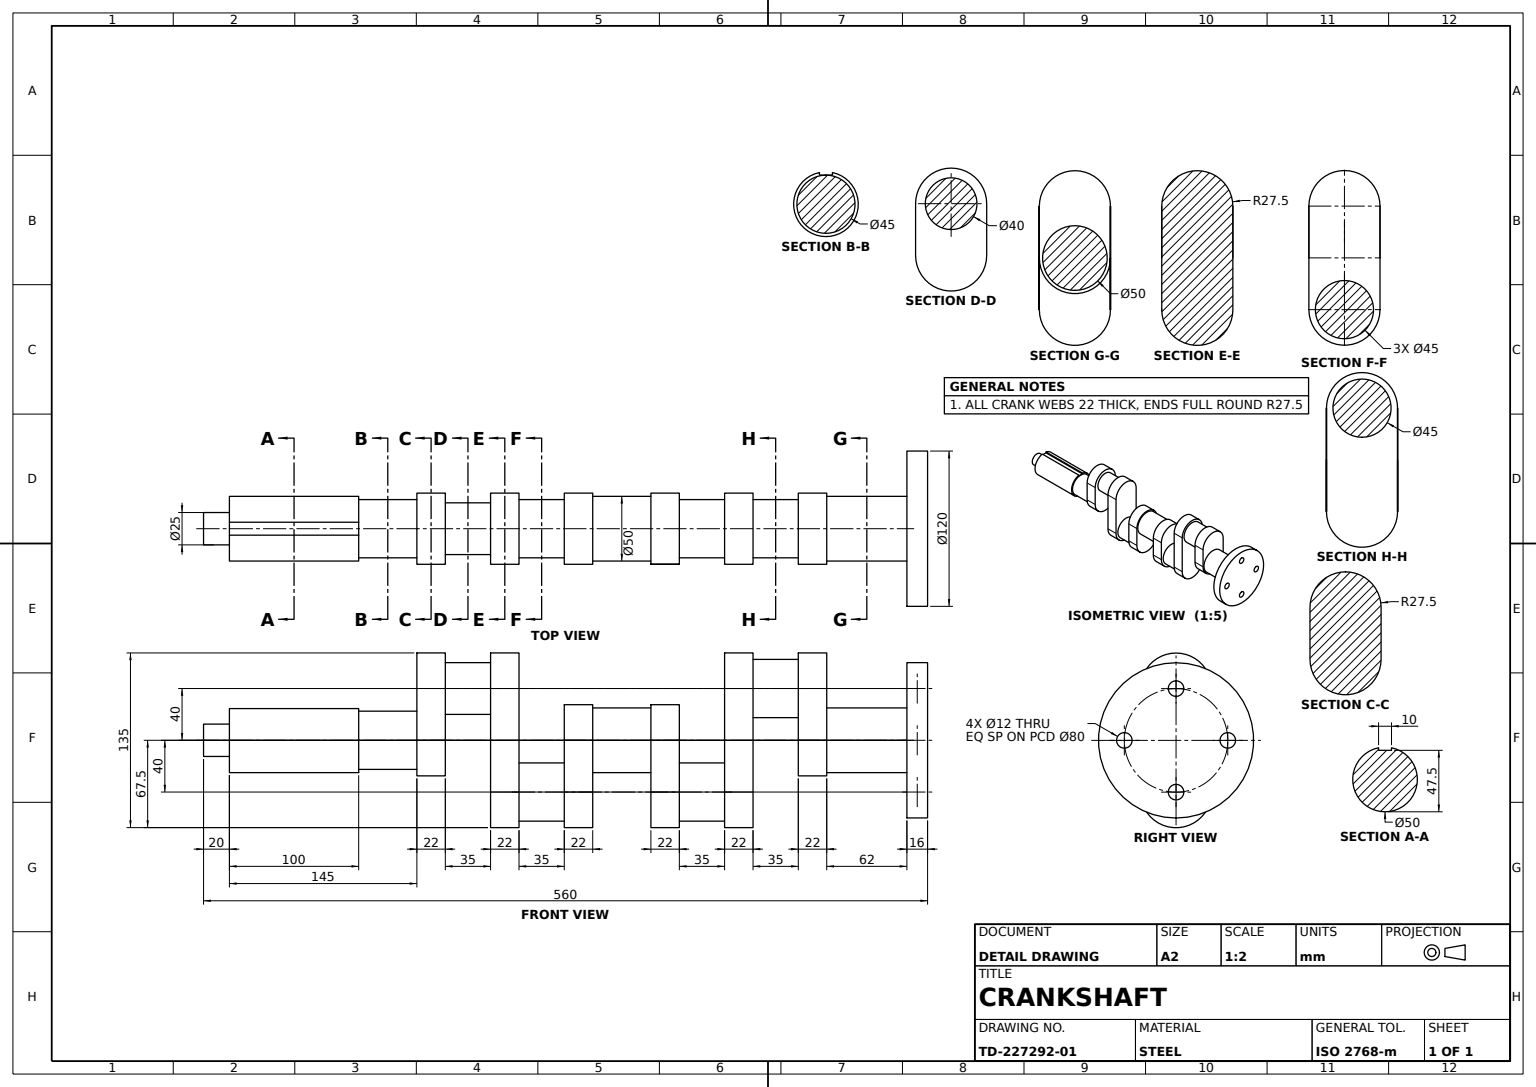
solid
v1 (-17.5,0,135)
v2 (-62.5,0,135)
e1 v1 v2 CIRCLE(AX(P(-40,0,135),D(0,0,1),D(1,0,0)),22.5)
e2 v2 v1 CIRCLE(AX(P(-40,0,135),D(0,0,1),D(1,0,0)),22.5)
v3 (-40,27.5,135)
v4 (-67.5,0,135)
e3 v3 v4 CIRCLE(AX(P(-40,0,135),D(0,0,1),D(1,0,0)),27.5)
v5 (40,27.5,135)
e4 v5 v3 LINE
v6 (40,-27.5,135)
e5 v6 v5 CIRCLE(AX(P(40,0,135),D(0,0,1),D(1,0,0)),27.5)
v7 (-40,-27.5,135)
e6 v7 v6 LINE
e7 v4 v7 CIRCLE(AX(P(-40,0,135),D(0,0,1),D(1,0,0)),27.5)
face PLANE(AX(P(-40,0,135),D(0,0,1),D(1,0,0))) rev [e1 e2] [-e3 -e4 -e5 -e6 -e7]
v8 (-6,40,0)
v9 (-6,40,16)
e8 v8 v9 LINE
v10 (6,40,16)
e9 v9 v10 CIRCLE(AX(P(0,40,16),D(0,0,1),D(1,0,0)),6)
v11 (6,40,0)
e10 v11 v10 LINE
e11 v8 v11 CIRCLE(AX(P(0,40,0),D(0,0,1),D(1,0,0)),6)
face CYL(AX(P(0,40,-4),D(0,0,1),D(1,0,0)),6) rev [e8 e9 -e10 -e11]
v12 (17.5,0,281)
v13 (62.5,0,281)
e12 v12 v13 CIRCLE(AX(P(40,0,281),D(0,0,1),D(1,0,0)),22.5)
e13 v13 v12 CIRCLE(AX(P(40,0,281),D(0,0,1),D(1,0,0)),22.5)
v14 (40,27.5,281)
v15 (0,27.5,281)
e14 v14 v15 LINE
v16 (-27.5,0,281)
e15 v15 v16 CIRCLE(AX(P(0,0,281),D(0,0,1),D(1,0,0)),27.5)
v17 (0,-27.5,281)
e16 v16 v17 CIRCLE(AX(P(0,0,281),D(0,0,1),D(1,0,0)),27.5)
v18 (40,-27.5,281)
e17 v17 v18 LINE
e18 v18 v14 CIRCLE(AX(P(40,0,281),D(0,0,1),D(1,0,0)),27.5)
face PLANE(AX(P(0,0,281),D(0,0,1),D(1,0,0))) [-e12 -e13] [e14 e15 e16 e17 e18]
v19 (12.5,0,540)
v20 (-12.5,0,540)
e19 v19 v20 CIRCLE(AX(P(0,0,540),D(0,0,1),D(1,0,0)),12.5)
e20 v20 v19 CIRCLE(AX(P(0,0,540),D(0,0,1),D(1,0,0)),12.5)
v21 (25,0,540)
v22 (-24.494897,5,540)
e21 v21 v22 CIRCLE(AX(P(0,0,540),D(0,0,1),D(1,0,0)),25)
v23 (-22.5,5,540)
e22 v23 v22 LINE
v24 (-22.5,-5,540)
e23 v24 v23 LINE
v25 (-24.494897,-5,540)
e24 v25 v24 LINE
e25 v25 v21 CIRCLE(AX(P(0,0,540),D(0,0,1),D(1,0,0)),25)
face PLANE(AX(P(0,0,540),D(0,0,1),D(1,0,0))) [-e19 -e20] [e21 -e22 -e23 -e24 e25]
v26 (40,27.5,338)
v27 (40,27.5,316)
e26 v26 v27 LINE
v28 (40,-27.5,338)
e27 v28 v26 CIRCLE(AX(P(40,0,338),D(0,0,1),D(1,0,0)),27.5)
v29 (40,-27.5,316)
e28 v28 v29 LINE
e29 v29 v27 CIRCLE(AX(P(40,0,316),D(0,0,1),D(1,0,0)),27.5)
face CYL(AX(P(40,0,338),D(0,0,-1),D(-1,0,0)),27.5) [-e26 -e27 e28 e29]
v30 (62.5,0,192)
v31 (62.5,0,157)
e30 v30 v31 LINE
v32 (17.5,0,192)
e31 v32 v30 CIRCLE(AX(P(40,0,192),D(0,0,1),D(1,0,0)),22.5)
v33 (17.5,0,157)
e32 v32 v33 LINE
e33 v33 v31 CIRCLE(AX(P(40,0,157),D(0,0,1),D(1,0,0)),22.5)
face CYL(AX(P(40,0,192),D(0,0,-1),D(-1,0,0)),22.5) [-e30 -e31 e32 e33]
v34 (12.5,0,560)
e34 v34 v19 LINE
v35 (-12.5,0,560)
e35 v35 v34 CIRCLE(AX(P(0,0,560),D(0,0,1),D(1,0,0)),12.5)
e36 v35 v20 LINE
face CYL(AX(P(0,0,560),D(0,0,-1),D(-1,0,0)),12.5) [e20 -e34 -e35 e36]
v36 (25,0,78)
v37 (-25,0,78)
e37 v36 v37 CIRCLE(AX(P(0,0,78),D(0,0,1),D(1,0,0)),25)
v38 (25,0,16)
e38 v36 v38 LINE
v39 (-25,0,16)
e39 v38 v39 CIRCLE(AX(P(0,0,16),D(0,0,1),D(1,0,0)),25)
e40 v37 v39 LINE
face CYL(AX(P(0,0,78),D(0,0,-1),D(-1,0,0)),25) [-e37 e38 e39 -e40]
v40 (-67.5,0,157)
e41 v40 v4 LINE
v41 (-40,27.5,157)
e42 v41 v40 CIRCLE(AX(P(-40,0,157),D(0,0,1),D(1,0,0)),27.5)
e43 v41 v3 LINE
face CYL(AX(P(-40,0,157),D(0,0,-1),D(-1,0,0)),27.5) [-e41 -e42 e43 e3]
v42 (-20,0,373)
v43 (-20,0,338)
e44 v42 v43 LINE
v44 (-60,0,338)
e45 v43 v44 CIRCLE(AX(P(-40,0,338),D(0,0,1),D(1,0,0)),20)
v45 (-60,0,373)
e46 v45 v44 LINE
e47 v42 v45 CIRCLE(AX(P(-40,0,373),D(0,0,1),D(1,0,0)),20)
face CYL(AX(P(-40,0,373),D(0,0,-1),D(-1,0,0)),20) [e44 e45 -e46 -e47]
v46 (-24.494897,-5,440)
e48 v46 v25 LINE
v47 (25,0,440)
e49 v46 v47 CIRCLE(AX(P(0,0,440),D(0,0,1),D(1,0,0)),25)
e50 v47 v21 LINE
face CYL(AX(P(0,0,440),D(0,0,1),D(1,0,0)),25) [-e25 -e48 e49 e50]
e51 v11 v8 CIRCLE(AX(P(0,40,0),D(0,0,1),D(1,0,0)),6)
e52 v10 v9 CIRCLE(AX(P(0,40,16),D(0,0,1),D(1,0,0)),6)
face CYL(AX(P(0,40,-4),D(0,0,1),D(1,0,0)),6) rev [-e8 -e51 e10 e52]
v48 (22.5,0,440)
v49 (-22.5,0,440)
e53 v48 v49 CIRCLE(AX(P(0,0,440),D(0,0,1),D(1,0,0)),22.5)
v50 (-22.5,5,440)
e54 v49 v50 LINE
v51 (-24.494897,5,440)
e55 v50 v51 LINE
e56 v47 v51 CIRCLE(AX(P(0,0,440),D(0,0,1),D(1,0,0)),25)
v52 (-22.5,-5,440)
e57 v46 v52 LINE
e58 v52 v49 LINE
e59 v49 v48 CIRCLE(AX(P(0,0,440),D(0,0,1),D(1,0,0)),22.5)
face PLANE(AX(P(0,0,440),D(0,0,1),D(1,0,0))) rev [e53 e54 e55 -e56 -e49 e57 e58 e59]
v53 (62.5,0,316)
e60 v53 v13 LINE
v54 (17.5,0,316)
e61 v54 v12 LINE
e62 v53 v54 CIRCLE(AX(P(40,0,316),D(0,0,1),D(1,0,0)),22.5)
face CYL(AX(P(40,0,316),D(0,0,-1),D(-1,0,0)),22.5) [e60 e13 -e61 -e62]
v55 (-40,27.5,338)
e63 v26 v55 LINE
v56 (-40,27.5,316)
e64 v27 v56 LINE
e65 v55 v56 LINE
face PLANE(AX(P(40,27.5,338),D(0,-1,0),D(1,0,0))) rev [-e63 e26 e64 -e65]
e66 v31 v33 CIRCLE(AX(P(40,0,157),D(0,0,1),D(1,0,0)),22.5)
e67 v30 v32 CIRCLE(AX(P(40,0,192),D(0,0,1),D(1,0,0)),22.5)
face CYL(AX(P(40,0,192),D(0,0,-1),D(-1,0,0)),22.5) [e30 e66 -e32 -e67]
v57 (0,27.5,395)
v58 (0,27.5,373)
e68 v57 v58 LINE
v59 (-40,27.5,373)
e69 v58 v59 LINE
v60 (-40,27.5,395)
e70 v60 v59 LINE
e71 v57 v60 LINE
face PLANE(AX(P(-40,27.5,395),D(0,-1,0),D(0,0,-1))) rev [e68 e69 -e70 -e71]
v61 (40,-27.5,157)
e72 v61 v6 LINE
v62 (40,27.5,157)
e73 v62 v5 LINE
e74 v61 v62 CIRCLE(AX(P(40,0,157),D(0,0,1),D(1,0,0)),27.5)
face CYL(AX(P(40,0,157),D(0,0,-1),D(-1,0,0)),27.5) [e72 e5 -e73 -e74]
e75 v50 v23 LINE
e76 v51 v22 LINE
face PLANE(AX(P(-24.494897,5,440),D(0,1,0),D(0,0,1))) rev [-e55 e75 e22 -e76]
v63 (-60,0,16)
v64 (60,0,16)
e77 v63 v64 CIRCLE(AX(P(0,0,16),D(0,0,1),D(1,0,0)),60)
v65 (-60,0,0)
e78 v63 v65 LINE
v66 (60,0,0)
e79 v65 v66 CIRCLE(AX(P(0,0,0),D(0,0,1),D(1,0,0)),60)
e80 v64 v66 LINE
face CYL(AX(P(0,0,16),D(0,0,-1),D(-1,0,0)),60) [-e77 e78 e79 -e80]
v67 (0,-27.5,214)
v68 (0,-27.5,192)
e81 v67 v68 LINE
v69 (40,-27.5,192)
e82 v68 v69 LINE
v70 (40,-27.5,214)
e83 v70 v69 LINE
e84 v67 v70 LINE
face PLANE(AX(P(40,-27.5,214),D(0,1,0),D(-1,0,0))) rev [e81 e82 -e83 -e84]
v71 (40,27.5,192)
e85 v69 v71 CIRCLE(AX(P(40,0,192),D(0,0,1),D(1,0,0)),27.5)
v72 (-27.5,0,192)
e86 v72 v68 CIRCLE(AX(P(0,0,192),D(0,0,1),D(1,0,0)),27.5)
v73 (0,27.5,192)
e87 v73 v72 CIRCLE(AX(P(0,0,192),D(0,0,1),D(1,0,0)),27.5)
e88 v71 v73 LINE
face PLANE(AX(P(40,0,192),D(0,0,1),D(1,0,0))) rev [e67 e31] [-e85 -e82 -e86 -e87 -e88]
v74 (-22.5,0,395)
e89 v49 v74 LINE
v75 (22.5,0,395)
e90 v74 v75 CIRCLE(AX(P(0,0,395),D(0,0,1),D(1,0,0)),22.5)
e91 v48 v75 LINE
face CYL(AX(P(0,0,540),D(0,0,-1),D(-1,0,0)),22.5) [e89 e90 -e91 -e59]
v76 (-6,-40,0)
v77 (-6,-40,16)
e92 v76 v77 LINE
v78 (6,-40,16)
e93 v77 v78 CIRCLE(AX(P(0,-40,16),D(0,0,1),D(1,0,0)),6)
v79 (6,-40,0)
e94 v79 v78 LINE
e95 v76 v79 CIRCLE(AX(P(0,-40,0),D(0,0,1),D(1,0,0)),6)
face CYL(AX(P(0,-40,-4),D(0,0,1),D(1,0,0)),6) rev [e92 e93 -e94 -e95]
v80 (-25,0,214)
v81 (25,0,214)
e96 v80 v81 CIRCLE(AX(P(0,0,214),D(0,0,1),D(1,0,0)),25)
v82 (25,0,259)
e97 v82 v81 LINE
v83 (-25,0,259)
e98 v83 v82 CIRCLE(AX(P(0,0,259),D(0,0,1),D(1,0,0)),25)
e99 v83 v80 LINE
face CYL(AX(P(0,0,259),D(0,0,-1),D(-1,0,0)),25) [e96 -e97 -e98 e99]
v84 (-62.5,0,100)
e100 v2 v84 LINE
v85 (-17.5,0,100)
e101 v84 v85 CIRCLE(AX(P(-40,0,100),D(0,0,1),D(1,0,0)),22.5)
e102 v1 v85 LINE
face CYL(AX(P(-40,0,135),D(0,0,-1),D(-1,0,0)),22.5) [-e2 e100 e101 -e102]
v86 (-46,0,0)
v87 (-46,0,16)
e103 v86 v87 LINE
v88 (-34,0,0)
e104 v88 v86 CIRCLE(AX(P(-40,0,0),D(0,0,1),D(1,0,0)),6)
v89 (-34,0,16)
e105 v88 v89 LINE
e106 v89 v87 CIRCLE(AX(P(-40,0,16),D(0,0,1),D(1,0,0)),6)
face CYL(AX(P(-40,0,-4),D(0,0,1),D(1,0,0)),6) rev [-e103 -e104 e105 e106]
v90 (-27.5,0,259)
e107 v16 v90 LINE
v91 (0,27.5,259)
e108 v15 v91 LINE
e109 v91 v90 CIRCLE(AX(P(0,0,259),D(0,0,1),D(1,0,0)),27.5)
face CYL(AX(P(0,0,281),D(0,0,-1),D(-1,0,0)),27.5) [-e107 -e15 e108 e109]
e110 v45 v42 CIRCLE(AX(P(-40,0,373),D(0,0,1),D(1,0,0)),20)
e111 v44 v43 CIRCLE(AX(P(-40,0,338),D(0,0,1),D(1,0,0)),20)
face CYL(AX(P(-40,0,373),D(0,0,-1),D(-1,0,0)),20) [-e110 e46 e111 -e44]
v92 (-40,-27.5,338)
e112 v92 v28 LINE
v93 (-67.5,0,338)
e113 v55 v93 CIRCLE(AX(P(-40,0,338),D(0,0,1),D(1,0,0)),27.5)
e114 v93 v92 CIRCLE(AX(P(-40,0,338),D(0,0,1),D(1,0,0)),27.5)
face PLANE(AX(P(40,0,338),D(0,0,1),D(1,0,0))) [-e45 -e111] [e112 e27 e63 e113 e114]
e115 v75 v74 CIRCLE(AX(P(0,0,395),D(0,0,1),D(1,0,0)),22.5)
face CYL(AX(P(0,0,540),D(0,0,-1),D(-1,0,0)),22.5) [e91 e115 -e89 -e53]
v94 (0,-27.5,395)
v95 (0,-27.5,373)
e116 v94 v95 LINE
v96 (-40,-27.5,395)
e117 v96 v94 LINE
v97 (-40,-27.5,373)
e118 v96 v97 LINE
e119 v97 v95 LINE
face PLANE(AX(P(-40,-27.5,395),D(0,1,0),D(0,0,1))) rev [-e116 -e117 e118 e119]
e120 v95 v58 CIRCLE(AX(P(0,0,373),D(0,0,1),D(1,0,0)),27.5)
e121 v94 v57 CIRCLE(AX(P(0,0,395),D(0,0,1),D(1,0,0)),27.5)
face CYL(AX(P(0,0,395),D(0,0,-1),D(-1,0,0)),27.5) [e120 -e68 -e121 e116]
e122 v54 v53 CIRCLE(AX(P(40,0,316),D(0,0,1),D(1,0,0)),22.5)
face CYL(AX(P(40,0,316),D(0,0,-1),D(-1,0,0)),22.5) [e12 -e60 -e122 e61]
v98 (-27.5,0,214)
e123 v98 v72 LINE
v99 (0,27.5,214)
e124 v99 v98 CIRCLE(AX(P(0,0,214),D(0,0,1),D(1,0,0)),27.5)
e125 v99 v73 LINE
face CYL(AX(P(0,0,214),D(0,0,-1),D(-1,0,0)),27.5) [-e123 -e124 e125 e87]
e126 v34 v35 CIRCLE(AX(P(0,0,560),D(0,0,1),D(1,0,0)),12.5)
face CYL(AX(P(0,0,560),D(0,0,-1),D(-1,0,0)),12.5) [-e126 e34 e19 -e36]
e127 v86 v88 CIRCLE(AX(P(-40,0,0),D(0,0,1),D(1,0,0)),6)
e128 v79 v76 CIRCLE(AX(P(0,-40,0),D(0,0,1),D(1,0,0)),6)
v100 (46,0,0)
v101 (34,0,0)
e129 v100 v101 CIRCLE(AX(P(40,0,0),D(0,0,1),D(1,0,0)),6)
e130 v101 v100 CIRCLE(AX(P(40,0,0),D(0,0,1),D(1,0,0)),6)
e131 v66 v65 CIRCLE(AX(P(0,0,0),D(0,0,1),D(1,0,0)),60)
face PLANE(AX(P(0,0,0),D(0,0,1),D(1,0,0))) rev [e11 e51] [e127 e104] [e95 e128] [e129 e130] [-e131 -e79]
v102 (-40,-27.5,316)
e132 v92 v102 LINE
e133 v102 v29 LINE
face PLANE(AX(P(40,-27.5,338),D(0,1,0),D(-1,0,0))) rev [-e112 e132 e133 -e28]
face PLANE(AX(P(0,0,560),D(0,0,1),D(1,0,0))) [e126 e35]
v103 (-67.5,0,316)
e134 v93 v103 LINE
e135 v56 v103 CIRCLE(AX(P(-40,0,316),D(0,0,1),D(1,0,0)),27.5)
face CYL(AX(P(-40,0,338),D(0,0,-1),D(-1,0,0)),27.5) [-e134 -e113 e65 e135]
e136 v85 v84 CIRCLE(AX(P(-40,0,100),D(0,0,1),D(1,0,0)),22.5)
face CYL(AX(P(-40,0,135),D(0,0,-1),D(-1,0,0)),22.5) [-e100 -e1 e102 e136]
e137 v52 v24 LINE
face PLANE(AX(P(-22.5,-5,440),D(1,0,0),D(0,0,-1))) rev [-e75 -e54 -e58 e137 e23]
face CYL(AX(P(0,0,440),D(0,0,1),D(1,0,0)),25) [e56 e76 -e21 -e50]
v104 (40,-27.5,259)
e138 v18 v104 LINE
v105 (0,-27.5,259)
e139 v17 v105 LINE
e140 v105 v104 LINE
face PLANE(AX(P(0,-27.5,281),D(0,1,0),D(0,0,1))) rev [-e138 -e17 e139 e140]
v106 (-67.5,0,373)
e141 v59 v106 CIRCLE(AX(P(-40,0,373),D(0,0,1),D(1,0,0)),27.5)
e142 v106 v97 CIRCLE(AX(P(-40,0,373),D(0,0,1),D(1,0,0)),27.5)
face PLANE(AX(P(-40,0,373),D(0,0,1),D(1,0,0))) rev [-e141 -e69 -e120 -e119 -e142] [e47 e110]
v107 (0,27.5,100)
v108 (0,27.5,78)
e143 v107 v108 LINE
v109 (0,-27.5,100)
e144 v109 v107 CIRCLE(AX(P(0,0,100),D(0,0,1),D(1,0,0)),27.5)
v110 (0,-27.5,78)
e145 v109 v110 LINE
e146 v110 v108 CIRCLE(AX(P(0,0,78),D(0,0,1),D(1,0,0)),27.5)
face CYL(AX(P(0,0,100),D(0,0,-1),D(-1,0,0)),27.5) [-e143 -e144 e145 e146]
e147 v81 v80 CIRCLE(AX(P(0,0,214),D(0,0,1),D(1,0,0)),25)
e148 v82 v83 CIRCLE(AX(P(0,0,259),D(0,0,1),D(1,0,0)),25)
face CYL(AX(P(0,0,259),D(0,0,-1),D(-1,0,0)),25) [e97 e147 -e99 -e148]
v111 (-67.5,0,395)
e149 v111 v96 CIRCLE(AX(P(-40,0,395),D(0,0,1),D(1,0,0)),27.5)
e150 v60 v111 CIRCLE(AX(P(-40,0,395),D(0,0,1),D(1,0,0)),27.5)
face PLANE(AX(P(-40,0,395),D(0,0,1),D(1,0,0))) [-e115 -e90] [e149 e117 e121 e71 e150]
e151 v103 v102 CIRCLE(AX(P(-40,0,316),D(0,0,1),D(1,0,0)),27.5)
face CYL(AX(P(-40,0,338),D(0,0,-1),D(-1,0,0)),27.5) [-e132 -e114 e134 e151]
v112 (40,27.5,214)
e152 v112 v71 LINE
e153 v112 v99 LINE
face PLANE(AX(P(40,27.5,214),D(0,-1,0),D(0,0,-1))) rev [e152 e88 -e125 -e153]
e154 v111 v106 LINE
face CYL(AX(P(-40,0,395),D(0,0,-1),D(-1,0,0)),27.5) [e154 e142 -e118 -e149]
e155 v62 v41 LINE
face PLANE(AX(P(-40,27.5,157),D(0,-1,0),D(1,0,0))) rev [e73 e4 -e43 -e155]
v113 (-67.5,0,100)
v114 (-40,-27.5,100)
e156 v113 v114 CIRCLE(AX(P(-40,0,100),D(0,0,1),D(1,0,0)),27.5)
v115 (-67.5,0,78)
e157 v113 v115 LINE
v116 (-40,-27.5,78)
e158 v115 v116 CIRCLE(AX(P(-40,0,78),D(0,0,1),D(1,0,0)),27.5)
e159 v114 v116 LINE
face CYL(AX(P(-40,0,100),D(0,0,-1),D(-1,0,0)),27.5) [-e156 e157 e158 -e159]
v117 (-40,-27.5,157)
e160 v40 v117 CIRCLE(AX(P(-40,0,157),D(0,0,1),D(1,0,0)),27.5)
e161 v117 v61 LINE
face PLANE(AX(P(-40,0,157),D(0,0,1),D(1,0,0))) [-e66 -e33] [e74 e155 e42 e160 e161]
e162 v114 v109 LINE
e163 v116 v110 LINE
face PLANE(AX(P(0,-27.5,100),D(0,1,0),D(0,0,1))) rev [-e162 e159 e163 -e145]
v118 (34,0,16)
e164 v101 v118 LINE
v119 (46,0,16)
e165 v118 v119 CIRCLE(AX(P(40,0,16),D(0,0,1),D(1,0,0)),6)
e166 v100 v119 LINE
face CYL(AX(P(40,0,-4),D(0,0,1),D(1,0,0)),6) rev [-e130 e164 e165 -e166]
face PLANE(AX(P(40,0,316),D(0,0,1),D(1,0,0))) rev [e122 e62] [-e133 -e151 -e135 -e64 -e29]
face CYL(AX(P(-40,0,395),D(0,0,-1),D(-1,0,0)),27.5) [e141 -e154 -e150 e70]
e167 v78 v77 CIRCLE(AX(P(0,-40,16),D(0,0,1),D(1,0,0)),6)
face CYL(AX(P(0,-40,-4),D(0,0,1),D(1,0,0)),6) rev [-e128 e94 e167 -e92]
v120 (40,27.5,259)
e168 v14 v120 LINE
e169 v120 v91 LINE
face PLANE(AX(P(0,27.5,281),D(0,-1,0),D(0,0,-1))) rev [-e108 -e14 e168 e169]
e170 v37 v36 CIRCLE(AX(P(0,0,78),D(0,0,1),D(1,0,0)),25)
v121 (-40,27.5,78)
e171 v121 v115 CIRCLE(AX(P(-40,0,78),D(0,0,1),D(1,0,0)),27.5)
e172 v108 v121 LINE
face PLANE(AX(P(0,0,78),D(0,0,1),D(1,0,0))) rev [e170 e37] [-e163 -e158 -e171 -e172 -e146]
e173 v39 v38 CIRCLE(AX(P(0,0,16),D(0,0,1),D(1,0,0)),25)
e174 v87 v89 CIRCLE(AX(P(-40,0,16),D(0,0,1),D(1,0,0)),6)
e175 v119 v118 CIRCLE(AX(P(40,0,16),D(0,0,1),D(1,0,0)),6)
e176 v64 v63 CIRCLE(AX(P(0,0,16),D(0,0,1),D(1,0,0)),60)
face PLANE(AX(P(0,0,16),D(0,0,1),D(1,0,0))) [-e173 -e39] [-e174 -e106] [-e175 -e165] [-e9 -e52] [-e93 -e167] [e77 e176]
face CYL(AX(P(0,0,78),D(0,0,-1),D(-1,0,0)),25) [-e38 -e170 e40 e173]
e177 v117 v7 LINE
face PLANE(AX(P(-40,-27.5,157),D(0,1,0),D(-1,0,0))) rev [-e72 -e161 e177 e6]
face CYL(AX(P(-40,0,157),D(0,0,-1),D(-1,0,0)),27.5) [e41 e7 -e177 -e160]
e178 v104 v120 CIRCLE(AX(P(40,0,259),D(0,0,1),D(1,0,0)),27.5)
face CYL(AX(P(40,0,281),D(0,0,-1),D(-1,0,0)),27.5) [-e18 e138 e178 -e168]
v122 (-40,27.5,100)
e179 v122 v121 LINE
e180 v122 v113 CIRCLE(AX(P(-40,0,100),D(0,0,1),D(1,0,0)),27.5)
face CYL(AX(P(-40,0,100),D(0,0,-1),D(-1,0,0)),27.5) [e179 e171 -e157 -e180]
e181 v90 v105 CIRCLE(AX(P(0,0,259),D(0,0,1),D(1,0,0)),27.5)
face PLANE(AX(P(0,0,259),D(0,0,1),D(1,0,0))) rev [-e140 -e181 -e109 -e169 -e178] [e98 e148]
face CYL(AX(P(0,0,281),D(0,0,-1),D(-1,0,0)),27.5) [e181 -e139 -e16 e107]
e182 v107 v122 LINE
face PLANE(AX(P(0,27.5,100),D(0,-1,0),D(1,0,0))) rev [e143 e172 -e179 -e182]
e183 v98 v67 CIRCLE(AX(P(0,0,214),D(0,0,1),D(1,0,0)),27.5)
face CYL(AX(P(0,0,214),D(0,0,-1),D(-1,0,0)),27.5) [e123 e86 -e81 -e183]
face PLANE(AX(P(-24.494897,-5,440),D(0,-1,0),D(0,0,-1))) rev [e24 -e137 -e57 e48]
face PLANE(AX(P(0,0,100),D(0,0,1),D(1,0,0))) [-e101 -e136] [e162 e144 e182 e180 e156]
e184 v70 v112 CIRCLE(AX(P(40,0,214),D(0,0,1),D(1,0,0)),27.5)
face CYL(AX(P(40,0,214),D(0,0,-1),D(-1,0,0)),27.5) [-e184 e83 e85 -e152]
face CYL(AX(P(0,0,16),D(0,0,-1),D(-1,0,0)),60) [-e78 -e176 e80 e131]
face PLANE(AX(P(40,0,214),D(0,0,1),D(1,0,0))) [-e147 -e96] [e84 e184 e153 e124 e183]
face CYL(AX(P(40,0,-4),D(0,0,1),D(1,0,0)),6) rev [-e129 e166 e175 -e164]
face CYL(AX(P(-40,0,-4),D(0,0,1),D(1,0,0)),6) rev [-e127 e103 e174 -e105]
